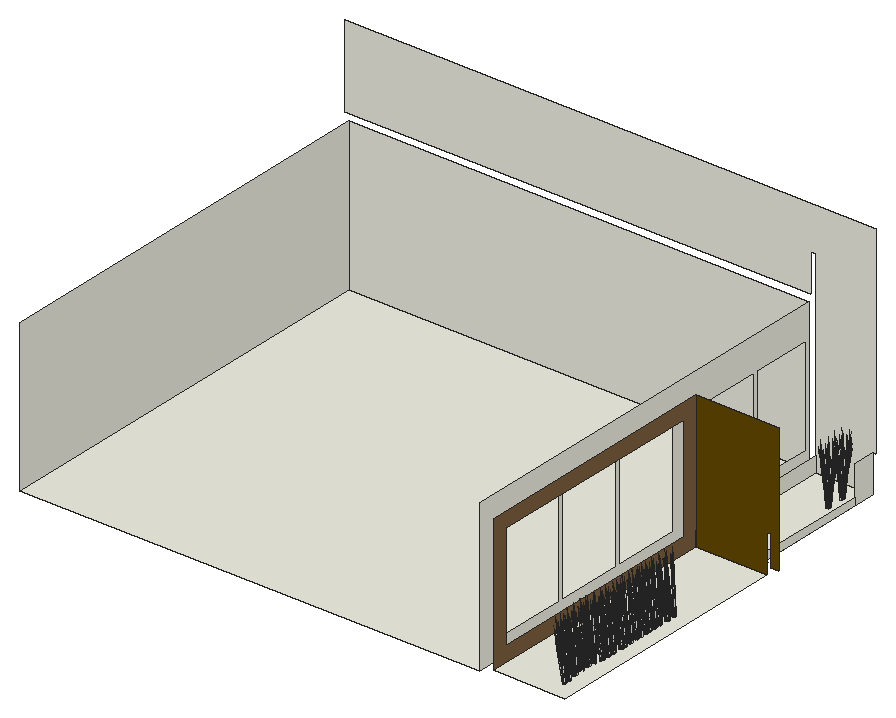
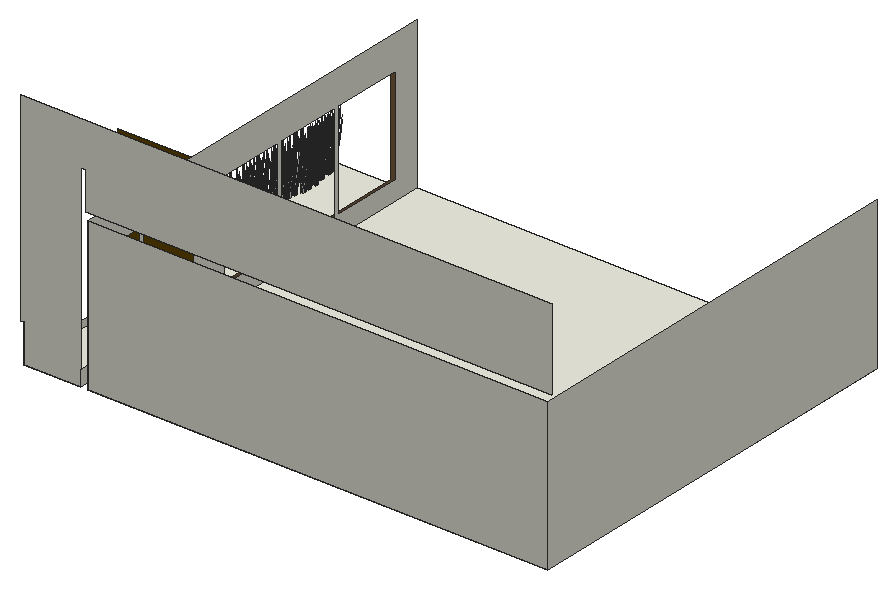
# SketchUp Ruby script. Lengths in inches.
U = 1.inch
M = Sketchup.active_model
def pt(a) = Geom::Point3d.new(a.map { |v| v * U })
def face(e, loops, mat)
  f = e.add_face(loops[0].map { |a| pt(a) })
  loops[1..].each { |l| e.add_face(l.map { |a| pt(a) }).erase! }
  f.material = f.back_material = mat if mat
  f
end
# faces: each face lists its corners as indices into pts; further lists are holes
def faces(e, pts, list, mat = nil) = list.each { |f| face(e, (f[0].is_a?(Array) ? f : [f]).map { |l| l.map { |i| pts[i] } }, mat) }
# xy, xz, yz: faces in a plane at the given z, y or x. An outline is a flat list of corners, or four numbers for a rectangle; further outlines are holes
def ring(l) = l.size == 4 ? [[l[0], l[1]], [l[2], l[1]], [l[2], l[3]], [l[0], l[3]]] : l.each_slice(2).to_a
def flat(e, list, mat, &to3) = list.each { |f| face(e, (f[0].is_a?(Array) ? f : [f]).map { |l| ring(l).map { |u, v| to3.(u, v) } }, mat) }
def xy(e, z, list, mat = nil) = flat(e, list, mat) { |x, y| [x, y, z] }
def xz(e, y, list, mat = nil) = flat(e, list, mat) { |x, z| [x, y, z] }
def yz(e, x, list, mat = nil) = flat(e, list, mat) { |y, z| [x, y, z] }
def lines(e, pts, list) = list.each { |a, b| e.add_line(pt(pts[a]), pt(pts[b])) }
# prism: a flat outline (further loops are holes) pulled along v
def prism(e, loops, v, mat = nil)
  f = face(e, loops, mat); d = Geom::Vector3d.new(v.map { |x| x * U })
  f.pushpull(f.normal.samedirection?(d) ? d.length : -d.length)
end
def box(e, o, s, mat = nil) = prism(e, [[o, [o[0] + s[0], o[1], o[2]], [o[0] + s[0], o[1] + s[1], o[2]], [o[0], o[1] + s[1], o[2]]]], [0, 0, s[2]], mat)
def at(x, y, z, deg = 0) = Geom::Transformation.translation(pt([x, y, z])) * Geom::Transformation.rotation(ORIGIN, Z_AXIS, deg.degrees)
def axes(o, x, y, z) = Geom::Transformation.new([*x, 0, *y, 0, *z, 0, *pt(o).to_a, 1])
def part(name) = M.definitions.add(name)
# library, detail: a bought-in or finely detailed component or shape, given as its bounding box
def library(name, o, s) = part(name).tap { |d| box(d.entities, o, s) }
def detail(e, o, s) = box(e.add_group.entities, o, s)
def put(e, d, t, mat = nil) = e.add_instance(d, t).tap { |i| i.material = mat if mat }
def group(e, t, mat = nil) = e.add_group.tap { |g| g.transformation = t; g.material = mat if mat }.entities
root = M.entities
M.materials.add("D01_Frost_White").color = [238, 238, 227]
M.materials.add("D08_Bronzed_Mustard").color = [102, 74, 0]
M.materials.add("LightPink_Translucent").color = [144, 107, 117]
M.materials["LightPink_Translucent"].alpha = 0.75
M.materials.add("Plywood_01_1K").color = [125, 96, 64]
c1 = part("blade")
p = [[2.15,0.21,22],[0,0.17,0],[0.09,0.45,0],[2.18,0.31,22],[2.29,0.31,22],[0.38,0.45,0],
  [2.48,0.24,33],[2.49,0.24,33],[2.48,0.22,33]]
faces(c1.entities,p,[[0,1,2,3],[4,5,2,3],[6,3,4,7],[8,0,3,6]])
c2 = part("seeds")
p = [[0.3,-0.1,1.38],[-0.01,-0.03,1.59],[-0.01,-0.03,0.03],[0.14,-0.07,-0.07],[0.29,-0.03,3],[0.15,0.01,3.11]]
faces(c2.entities,p,[[0,1,2,3],[1,0,4,5]],"LightPink_Translucent")
c3 = part("blade with seeds")
put(c3.entities,c1,at(0,0,0))
put(c3.entities,c2,axes([2.4,0.25,30.99],[1.5799,-0.05474,1.17369],[-0.12525,1.92788,0.29478],[-0.07173,-0.02425,1.56792]))
xy(root,150,[[10,367,376,694],[382,373,439,574.02],[382,574.02,430,586],[382,586,427,694]],"D01_Frost_White")
xz(root,574.02,[[382,150,439,150,439,180,442,180,442,156,448,156,448,258,382,258]],"D08_Bronzed_Mustard")
xz(root,694,[[382,150,427,150,427,180,430,180,430,341,7,341,7,276,377.5,276,377.5,306,382,306],[10,150,376,270]],"D01_Frost_White")
yz(root,10,[[367,150,694,270]],"D01_Frost_White")
yz(root,376,[[[367,150,694,270],[388,165,445.01,243],[505.01,165,559.02,243],[448.01,165,502.01,243],[589,165,640,243],[643,165,691,243]]],"D01_Frost_White")
yz(root,382,[[574.02,150,586,162],[586,150,694,162]],"D01_Frost_White")
yz(root,382,[[[373,150,574.02,258],[385,162,562.02,246]]],"Plywood_01_1K")
yz(root,427,[[586,150,676,156],[676,150,694,180]],"D01_Frost_White")
put(root,c3,axes([416.51,662.93,151.74],[-0.42629,-0.07733,-0.52676],[0.08996,-0.47699,-0.13825],[-0.12722,-0.0578,1.16273]))
put(root,c3,axes([416.51,676.81,151.74],[-0.42629,-0.07733,-0.52676],[0.08996,-0.47699,-0.13825],[-0.12722,-0.0578,1.16273]))
put(root,c3,axes([415.96,663.83,151.7],[-0.38354,-0.23583,-0.41945],[0.22925,-0.42288,0],[-0.08735,-0.05371,1.33059]))
put(root,c3,axes([415.96,677.71,151.7],[-0.38354,-0.23583,-0.41945],[0.22925,-0.42288,0],[-0.08735,-0.05371,1.33059]))
put(root,c3,axes([416.0625,663.66,151.71],[-0.09626,-0.41098,-0.2617],[0.38233,-0.1167,0.2617],[-0.07708,-0.04739,1.17405]))
put(root,c3,axes([416.0625,677.54,151.71],[-0.09626,-0.41098,-0.2617],[0.38233,-0.1167,0.2617],[-0.07708,-0.04739,1.17405]))
put(root,c3,axes([417.27,663.34,151.74],[-0.27603,0.35451,-0.52676],[-0.34289,-0.32147,-0.13825],[-0.11061,0.08844,1.16273]))
put(root,c3,axes([417.27,677.22,151.74],[-0.27603,0.35451,-0.52676],[-0.34289,-0.32147,-0.13825],[-0.11061,0.08844,1.16273]))
put(root,c3,axes([416.74,662.78,151.87],[-0.24618,-0.39589,-0.37796],[0.37289,-0.27878,0.1819],[-0.07967,-0.04899,1.2135]))
put(root,c3,axes([416.74,676.66,151.87],[-0.24618,-0.39589,-0.37796],[0.37289,-0.27878,0.1819],[-0.07967,-0.04899,1.2135]))
put(root,c3,axes([417.26,663.0625,151.87],[-0.44501,0.02912,-0.37796],[-0.04024,-0.48332,0.1819],[-0.07967,0.04899,1.2135]))
put(root,c3,axes([417.26,676.94,151.87],[-0.44501,0.02912,-0.37796],[-0.04024,-0.48332,0.1819],[-0.07967,0.04899,1.2135]))
put(root,c3,axes([417.73,664.3125,151.7],[-0.38354,0.23583,-0.41945],[-0.22925,-0.42288,0],[-0.08735,0.05371,1.33059]))
put(root,c3,axes([417.73,678.1875,151.7],[-0.38354,0.23583,-0.41945],[-0.22925,-0.42288,0],[-0.08735,0.05371,1.33059]))
put(root,c3,axes([415.46,661.96,151.7],[0,-0.47166,-0.41945],[0.45849,0,0],[0,-0.10742,1.33059]))
put(root,c3,axes([415.46,675.84,151.7],[0,-0.47166,-0.41945],[0.45849,0,0],[0,-0.10742,1.33059]))
put(root,c3,axes([417.64,664.125,151.71],[-0.38233,-0.1167,-0.2617],[0.09626,-0.41098,0.2617],[-0.07708,0.04739,1.17405]))
put(root,c3,axes([417.64,678,151.71],[-0.38233,-0.1167,-0.2617],[0.09626,-0.41098,0.2617],[-0.07708,0.04739,1.17405]))
put(root,c3,axes([416.45,662.03,151.77],[-0.1683,-0.48366,-0.58997],[0.48479,-0.17419,-0.15484],[-0.0186,-0.16378,1.30225]))
put(root,c3,axes([416.45,675.91,151.77],[-0.1683,-0.48366,-0.58997],[0.48479,-0.17419,-0.15484],[-0.0186,-0.16378,1.30225]))
put(root,c3,axes([415.65,661.97,151.71],[0.28606,-0.29428,-0.2617],[0.28606,0.29428,0.2617],[0,-0.09479,1.17405]))
put(root,c3,axes([415.65,675.85,151.71],[0.28606,-0.29428,-0.2617],[0.28606,0.29428,0.2617],[0,-0.09479,1.17405]))
put(root,c3,axes([416.7,662.15,151.87],[0.19883,-0.425,-0.37796],[0.41314,0.20454,0.1819],[0,-0.09797,1.2135]))
put(root,c3,axes([416.7,676.03,151.87],[0.19883,-0.425,-0.37796],[0.41314,0.20454,0.1819],[0,-0.09797,1.2135]))
put(root,c3,axes([417.75,662.72,151.87],[-0.19883,0.425,-0.37796],[-0.41314,-0.20454,0.1819],[0,0.09797,1.2135]))
put(root,c3,axes([417.75,676.6,151.87],[-0.19883,0.425,-0.37796],[-0.41314,-0.20454,0.1819],[0,0.09797,1.2135]))
put(root,c3,axes([418.8,662.9,151.71],[-0.28606,0.29428,-0.2617],[-0.28606,-0.29428,0.2617],[0,0.09479,1.17405]))
put(root,c3,axes([418.8,676.78,151.71],[-0.28606,0.29428,-0.2617],[-0.28606,-0.29428,0.2617],[0,0.09479,1.17405]))
put(root,c3,axes([417.99,662.85,151.77],[0.15027,0.43184,-0.5847],[-0.43285,0.15553,-0.15346],[0.01661,0.14623,1.29063]))
put(root,c3,axes([417.99,676.73,151.77],[0.15027,0.43184,-0.5847],[-0.43285,0.15553,-0.15346],[0.01661,0.14623,1.29063]))
put(root,c3,axes([416.82,660.75,151.71],[0.38233,0.1167,-0.2617],[-0.09626,0.41098,0.2617],[0.07708,-0.04739,1.17405]))
put(root,c3,axes([416.82,674.63,151.71],[0.38233,0.1167,-0.2617],[-0.09626,0.41098,0.2617],[0.07708,-0.04739,1.17405]))
put(root,c3,axes([419,662.92,151.7],[0,0.47166,-0.41945],[-0.45849,0,0],[0,0.10742,1.33059]))
put(root,c3,axes([419,676.79,151.7],[0,0.47166,-0.41945],[-0.45849,0,0],[0,0.10742,1.33059]))
put(root,c3,axes([416.73,660.57,151.7],[0.38354,-0.23583,-0.41945],[0.22925,0.42288,0],[0.08735,-0.05371,1.33059]))
put(root,c3,axes([416.73,674.44,151.7],[0.38354,-0.23583,-0.41945],[0.22925,0.42288,0],[0.08735,-0.05371,1.33059]))
put(root,c3,axes([417.72,662.1,151.87],[0.24618,0.39589,-0.37796],[-0.37289,0.27878,0.1819],[0.07967,0.04899,1.2135]))
put(root,c3,axes([417.72,675.97,151.87],[0.24618,0.39589,-0.37796],[-0.37289,0.27878,0.1819],[0.07967,0.04899,1.2135]))
put(root,c3,axes([417.19,661.53,151.74],[0.27603,-0.35451,-0.52676],[0.34289,0.32147,-0.13825],[0.11061,-0.08844,1.16273]))
put(root,c3,axes([417.19,675.41,151.74],[0.27603,-0.35451,-0.52676],[0.34289,0.32147,-0.13825],[0.11061,-0.08844,1.16273]))
put(root,c3,axes([418.4,661.22,151.71],[0.09626,0.41098,-0.2617],[-0.38233,0.1167,0.2617],[0.07708,0.04739,1.17405]))
put(root,c3,axes([418.4,675.1,151.71],[0.09626,0.41098,-0.2617],[-0.38233,0.1167,0.2617],[0.07708,0.04739,1.17405]))
put(root,c3,axes([418.5,661.04,151.7],[0.38354,0.23583,-0.41945],[-0.22925,0.42288,0],[0.08735,0.05371,1.33059]))
put(root,c3,axes([418.5,674.92,151.7],[0.38354,0.23583,-0.41945],[-0.22925,0.42288,0],[0.08735,0.05371,1.33059]))
put(root,c3,axes([417.94,661.95,151.74],[0.42629,0.07733,-0.52676],[-0.08996,0.47699,-0.13825],[0.12722,0.0578,1.16273]))
put(root,c3,axes([417.94,675.82,151.74],[0.42629,0.07733,-0.52676],[-0.08996,0.47699,-0.13825],[0.12722,0.0578,1.16273]))
put(root,c3,axes([426.07,405.04,151.74],[-0.42629,-0.07733,-0.52676],[0.08996,-0.47699,-0.13825],[-0.12722,-0.0578,1.16273]))
put(root,c3,axes([426.15,416.97,151.74],[-0.42629,-0.07733,-0.52676],[0.08996,-0.47699,-0.13825],[-0.12722,-0.0578,1.16273]))
put(root,c3,axes([426.22,411.59,151.74],[-0.42629,-0.07733,-0.52676],[0.08996,-0.47699,-0.13825],[-0.12722,-0.0578,1.16273]))
put(root,c3,axes([425.51,405.94,151.7],[-0.38354,-0.23583,-0.41945],[0.22925,-0.42288,0],[-0.08735,-0.05371,1.33059]))
put(root,c3,axes([425.59,417.875,151.7],[-0.38354,-0.23583,-0.41945],[0.22925,-0.42288,0],[-0.08735,-0.05371,1.33059]))
put(root,c3,axes([425.66,412.49,151.7],[-0.38354,-0.23583,-0.41945],[0.22925,-0.42288,0],[-0.08735,-0.05371,1.33059]))
put(root,c3,axes([425.62,405.77,151.71],[-0.09626,-0.41098,-0.2617],[0.38233,-0.1167,0.2617],[-0.07708,-0.04739,1.17405]))
put(root,c3,axes([425.69,417.7,151.71],[-0.09626,-0.41098,-0.2617],[0.38233,-0.1167,0.2617],[-0.07708,-0.04739,1.17405]))
put(root,c3,axes([427.16,397.46,151.74],[-0.42629,-0.07733,-0.52676],[0.08996,-0.47699,-0.13825],[-0.12722,-0.0578,1.16273]))
put(root,c3,axes([425.76,412.32,151.71],[-0.09626,-0.41098,-0.2617],[0.38233,-0.1167,0.2617],[-0.07708,-0.04739,1.17405]))
put(root,c3,axes([426.83,405.45,151.74],[-0.27603,0.35451,-0.52676],[-0.34289,-0.32147,-0.13825],[-0.11061,0.08844,1.16273]))
put(root,c3,axes([426.91,417.38,151.74],[-0.27603,0.35451,-0.52676],[-0.34289,-0.32147,-0.13825],[-0.11061,0.08844,1.16273]))
put(root,c3,axes([426.98,412,151.74],[-0.27603,0.35451,-0.52676],[-0.34289,-0.32147,-0.13825],[-0.11061,0.08844,1.16273]))
put(root,c3,axes([426.6,398.36,151.7],[-0.38354,-0.23583,-0.41945],[0.22925,-0.42288,0],[-0.08735,-0.05371,1.33059]))
put(root,c3,axes([426.29,404.89,151.87],[-0.24618,-0.39589,-0.37796],[0.37289,-0.27878,0.1819],[-0.07967,-0.04899,1.2135]))
put(root,c3,axes([426.37,416.82,151.87],[-0.24618,-0.39589,-0.37796],[0.37289,-0.27878,0.1819],[-0.07967,-0.04899,1.2135]))
put(root,c3,axes([426.4375,411.4375,151.87],[-0.24618,-0.39589,-0.37796],[0.37289,-0.27878,0.1819],[-0.07967,-0.04899,1.2135]))
put(root,c3,axes([426.82,405.17,151.87],[-0.44501,0.02912,-0.37796],[-0.04024,-0.48332,0.1819],[-0.07967,0.04899,1.2135]))
put(root,c3,axes([426.89,417.1,151.87],[-0.44501,0.02912,-0.37796],[-0.04024,-0.48332,0.1819],[-0.07967,0.04899,1.2135]))
put(root,c3,axes([426.96,411.72,151.87],[-0.44501,0.02912,-0.37796],[-0.04024,-0.48332,0.1819],[-0.07967,0.04899,1.2135]))
put(root,c3,axes([427.29,406.42,151.7],[-0.38354,0.23583,-0.41945],[-0.22925,-0.42288,0],[-0.08735,0.05371,1.33059]))
put(root,c3,axes([425.02,404.07,151.7],[0,-0.47166,-0.41945],[0.45849,0,0],[0,-0.10742,1.33059]))
put(root,c3,axes([427.36,418.35,151.7],[-0.38354,0.23583,-0.41945],[-0.22925,-0.42288,0],[-0.08735,0.05371,1.33059]))
put(root,c3,axes([425.09,416,151.7],[0,-0.47166,-0.41945],[0.45849,0,0],[0,-0.10742,1.33059]))
put(root,c3,axes([427.43,412.97,151.7],[-0.38354,0.23583,-0.41945],[-0.22925,-0.42288,0],[-0.08735,0.05371,1.33059]))
put(root,c3,axes([426.71,398.1875,151.71],[-0.09626,-0.41098,-0.2617],[0.38233,-0.1167,0.2617],[-0.07708,-0.04739,1.17405]))
put(root,c3,axes([425.16,410.62,151.7],[0,-0.47166,-0.41945],[0.45849,0,0],[0,-0.10742,1.33059]))
put(root,c3,axes([427.2,406.23,151.71],[-0.38233,-0.1167,-0.2617],[0.09626,-0.41098,0.2617],[-0.07708,0.04739,1.17405]))
put(root,c3,axes([427.27,418.16,151.71],[-0.38233,-0.1167,-0.2617],[0.09626,-0.41098,0.2617],[-0.07708,0.04739,1.17405]))
put(root,c3,axes([427.34,412.78,151.71],[-0.38233,-0.1167,-0.2617],[0.09626,-0.41098,0.2617],[-0.07708,0.04739,1.17405]))
put(root,c3,axes([427.92,397.875,151.74],[-0.27603,0.35451,-0.52676],[-0.34289,-0.32147,-0.13825],[-0.11061,0.08844,1.16273]))
put(root,c3,axes([426.01,404.14,151.77],[-0.1683,-0.48366,-0.58997],[0.48479,-0.17419,-0.15484],[-0.0186,-0.16378,1.30225]))
put(root,c3,axes([426.08,416.07,151.77],[-0.1683,-0.48366,-0.58997],[0.48479,-0.17419,-0.15484],[-0.0186,-0.16378,1.30225]))
put(root,c3,axes([428.51,384.47,151.74],[-0.42629,-0.07733,-0.52676],[0.08996,-0.47699,-0.13825],[-0.12722,-0.0578,1.16273]))
put(root,c3,axes([428.51,389.04,151.74],[-0.42629,-0.07733,-0.52676],[0.08996,-0.47699,-0.13825],[-0.12722,-0.0578,1.16273]))
put(root,c3,axes([428.51,423.125,151.74],[-0.42629,-0.07733,-0.52676],[0.08996,-0.47699,-0.13825],[-0.12722,-0.0578,1.16273]))
put(root,c3,axes([428.51,429.24,151.74],[-0.42629,-0.07733,-0.52676],[0.08996,-0.47699,-0.13825],[-0.12722,-0.0578,1.16273]))
put(root,c3,axes([428.51,434.15,151.74],[-0.42629,-0.07733,-0.52676],[0.08996,-0.47699,-0.13825],[-0.12722,-0.0578,1.16273]))
put(root,c3,axes([428.51,441.41,151.74],[-0.42629,-0.07733,-0.52676],[0.08996,-0.47699,-0.13825],[-0.12722,-0.0578,1.16273]))
put(root,c3,axes([428.51,445.1,151.74],[-0.42629,-0.07733,-0.52676],[0.08996,-0.47699,-0.13825],[-0.12722,-0.0578,1.16273]))
put(root,c3,axes([428.51,450.52,151.74],[-0.42629,-0.07733,-0.52676],[0.08996,-0.47699,-0.13825],[-0.12722,-0.0578,1.16273]))
put(root,c3,axes([428.51,457,151.74],[-0.42629,-0.07733,-0.52676],[0.08996,-0.47699,-0.13825],[-0.12722,-0.0578,1.16273]))
put(root,c3,axes([428.51,460.55,151.74],[-0.42629,-0.07733,-0.52676],[0.08996,-0.47699,-0.13825],[-0.12722,-0.0578,1.16273]))
put(root,c3,axes([428.51,465.95,151.74],[-0.42629,-0.07733,-0.52676],[0.08996,-0.47699,-0.13825],[-0.12722,-0.0578,1.16273]))
put(root,c3,axes([428.51,470.01,151.74],[-0.42629,-0.07733,-0.52676],[0.08996,-0.47699,-0.13825],[-0.12722,-0.0578,1.16273]))
put(root,c3,axes([428.51,474.33,151.74],[-0.42629,-0.07733,-0.52676],[0.08996,-0.47699,-0.13825],[-0.12722,-0.0578,1.16273]))
put(root,c3,axes([428.51,479.87,151.74],[-0.42629,-0.07733,-0.52676],[0.08996,-0.47699,-0.13825],[-0.12722,-0.0578,1.16273]))
put(root,c3,axes([428.51,487.08,151.74],[-0.42629,-0.07733,-0.52676],[0.08996,-0.47699,-0.13825],[-0.12722,-0.0578,1.16273]))
put(root,c3,axes([428.51,493.25,151.74],[-0.42629,-0.07733,-0.52676],[0.08996,-0.47699,-0.13825],[-0.12722,-0.0578,1.16273]))
put(root,c3,axes([427.38,397.31,151.87],[-0.24618,-0.39589,-0.37796],[0.37289,-0.27878,0.1819],[-0.07967,-0.04899,1.2135]))
put(root,c3,axes([426.15,410.6875,151.77],[-0.1683,-0.48366,-0.58997],[0.48479,-0.17419,-0.15484],[-0.0186,-0.16378,1.30225]))
put(root,c3,axes([425.21,404.08,151.71],[0.28606,-0.29428,-0.2617],[0.28606,0.29428,0.2617],[0,-0.09479,1.17405]))
put(root,c3,axes([425.29,416.01,151.71],[0.28606,-0.29428,-0.2617],[0.28606,0.29428,0.2617],[0,-0.09479,1.17405]))
put(root,c3,axes([427.9,397.59,151.87],[-0.44501,0.02912,-0.37796],[-0.04024,-0.48332,0.1819],[-0.07967,0.04899,1.2135]))
put(root,c3,axes([425.36,410.63,151.71],[0.28606,-0.29428,-0.2617],[0.28606,0.29428,0.2617],[0,-0.09479,1.17405]))
put(root,c3,axes([427.96,385.37,151.7],[-0.38354,-0.23583,-0.41945],[0.22925,-0.42288,0],[-0.08735,-0.05371,1.33059]))
put(root,c3,axes([427.96,389.9375,151.7],[-0.38354,-0.23583,-0.41945],[0.22925,-0.42288,0],[-0.08735,-0.05371,1.33059]))
put(root,c3,axes([427.96,424.03,151.7],[-0.38354,-0.23583,-0.41945],[0.22925,-0.42288,0],[-0.08735,-0.05371,1.33059]))
put(root,c3,axes([427.96,430.14,151.7],[-0.38354,-0.23583,-0.41945],[0.22925,-0.42288,0],[-0.08735,-0.05371,1.33059]))
put(root,c3,axes([427.96,435.05,151.7],[-0.38354,-0.23583,-0.41945],[0.22925,-0.42288,0],[-0.08735,-0.05371,1.33059]))
put(root,c3,axes([427.96,442.31,151.7],[-0.38354,-0.23583,-0.41945],[0.22925,-0.42288,0],[-0.08735,-0.05371,1.33059]))
put(root,c3,axes([427.96,446,151.7],[-0.38354,-0.23583,-0.41945],[0.22925,-0.42288,0],[-0.08735,-0.05371,1.33059]))
put(root,c3,axes([427.96,451.42,151.7],[-0.38354,-0.23583,-0.41945],[0.22925,-0.42288,0],[-0.08735,-0.05371,1.33059]))
put(root,c3,axes([427.96,457.91,151.7],[-0.38354,-0.23583,-0.41945],[0.22925,-0.42288,0],[-0.08735,-0.05371,1.33059]))
put(root,c3,axes([427.96,461.45,151.7],[-0.38354,-0.23583,-0.41945],[0.22925,-0.42288,0],[-0.08735,-0.05371,1.33059]))
put(root,c3,axes([427.96,466.86,151.7],[-0.38354,-0.23583,-0.41945],[0.22925,-0.42288,0],[-0.08735,-0.05371,1.33059]))
put(root,c3,axes([427.96,470.91,151.7],[-0.38354,-0.23583,-0.41945],[0.22925,-0.42288,0],[-0.08735,-0.05371,1.33059]))
put(root,c3,axes([427.96,475.23,151.7],[-0.38354,-0.23583,-0.41945],[0.22925,-0.42288,0],[-0.08735,-0.05371,1.33059]))
put(root,c3,axes([427.96,480.77,151.7],[-0.38354,-0.23583,-0.41945],[0.22925,-0.42288,0],[-0.08735,-0.05371,1.33059]))
put(root,c3,axes([427.96,487.98,151.7],[-0.38354,-0.23583,-0.41945],[0.22925,-0.42288,0],[-0.08735,-0.05371,1.33059]))
put(root,c3,axes([427.96,494.15,151.7],[-0.38354,-0.23583,-0.41945],[0.22925,-0.42288,0],[-0.08735,-0.05371,1.33059]))
put(root,c3,axes([428.37,398.84,151.7],[-0.38354,0.23583,-0.41945],[-0.22925,-0.42288,0],[-0.08735,0.05371,1.33059]))
put(root,c3,axes([426.1,396.49,151.7],[0,-0.47166,-0.41945],[0.45849,0,0],[0,-0.10742,1.33059]))
put(root,c3,axes([428.28,398.65,151.71],[-0.38233,-0.1167,-0.2617],[0.09626,-0.41098,0.2617],[-0.07708,0.04739,1.17405]))
put(root,c3,axes([428.0625,385.19,151.71],[-0.09626,-0.41098,-0.2617],[0.38233,-0.1167,0.2617],[-0.07708,-0.04739,1.17405]))
put(root,c3,axes([428.0625,389.76,151.71],[-0.09626,-0.41098,-0.2617],[0.38233,-0.1167,0.2617],[-0.07708,-0.04739,1.17405]))
put(root,c3,axes([428.0625,423.85,151.71],[-0.09626,-0.41098,-0.2617],[0.38233,-0.1167,0.2617],[-0.07708,-0.04739,1.17405]))
put(root,c3,axes([428.0625,429.97,151.71],[-0.09626,-0.41098,-0.2617],[0.38233,-0.1167,0.2617],[-0.07708,-0.04739,1.17405]))
put(root,c3,axes([428.0625,434.88,151.71],[-0.09626,-0.41098,-0.2617],[0.38233,-0.1167,0.2617],[-0.07708,-0.04739,1.17405]))
put(root,c3,axes([428.0625,442.13,151.71],[-0.09626,-0.41098,-0.2617],[0.38233,-0.1167,0.2617],[-0.07708,-0.04739,1.17405]))
put(root,c3,axes([428.0625,445.83,151.71],[-0.09626,-0.41098,-0.2617],[0.38233,-0.1167,0.2617],[-0.07708,-0.04739,1.17405]))
put(root,c3,axes([428.0625,451.25,151.71],[-0.09626,-0.41098,-0.2617],[0.38233,-0.1167,0.2617],[-0.07708,-0.04739,1.17405]))
put(root,c3,axes([428.0625,457.73,151.71],[-0.09626,-0.41098,-0.2617],[0.38233,-0.1167,0.2617],[-0.07708,-0.04739,1.17405]))
put(root,c3,axes([428.0625,461.28,151.71],[-0.09626,-0.41098,-0.2617],[0.38233,-0.1167,0.2617],[-0.07708,-0.04739,1.17405]))
put(root,c3,axes([428.0625,466.68,151.71],[-0.09626,-0.41098,-0.2617],[0.38233,-0.1167,0.2617],[-0.07708,-0.04739,1.17405]))
put(root,c3,axes([428.0625,470.73,151.71],[-0.09626,-0.41098,-0.2617],[0.38233,-0.1167,0.2617],[-0.07708,-0.04739,1.17405]))
put(root,c3,axes([428.0625,475.06,151.71],[-0.09626,-0.41098,-0.2617],[0.38233,-0.1167,0.2617],[-0.07708,-0.04739,1.17405]))
put(root,c3,axes([428.0625,480.59,151.71],[-0.09626,-0.41098,-0.2617],[0.38233,-0.1167,0.2617],[-0.07708,-0.04739,1.17405]))
put(root,c3,axes([428.0625,487.81,151.71],[-0.09626,-0.41098,-0.2617],[0.38233,-0.1167,0.2617],[-0.07708,-0.04739,1.17405]))
put(root,c3,axes([428.0625,493.97,151.71],[-0.09626,-0.41098,-0.2617],[0.38233,-0.1167,0.2617],[-0.07708,-0.04739,1.17405]))
put(root,c3,axes([427.09,396.56,151.77],[-0.1683,-0.48366,-0.58997],[0.48479,-0.17419,-0.15484],[-0.0186,-0.16378,1.30225]))
put(root,c3,axes([426.26,404.26,151.87],[0.19883,-0.425,-0.37796],[0.41314,0.20454,0.1819],[0,-0.09797,1.2135]))
put(root,c3,axes([426.34,416.19,151.87],[0.19883,-0.425,-0.37796],[0.41314,0.20454,0.1819],[0,-0.09797,1.2135]))
put(root,c3,axes([426.3,396.5,151.71],[0.28606,-0.29428,-0.2617],[0.28606,0.29428,0.2617],[0,-0.09479,1.17405]))
put(root,c3,axes([426.41,410.8125,151.87],[0.19883,-0.425,-0.37796],[0.41314,0.20454,0.1819],[0,-0.09797,1.2135]))
put(root,c3,axes([429.27,384.88,151.74],[-0.27603,0.35451,-0.52676],[-0.34289,-0.32147,-0.13825],[-0.11061,0.08844,1.16273]))
put(root,c3,axes([429.27,389.45,151.74],[-0.27603,0.35451,-0.52676],[-0.34289,-0.32147,-0.13825],[-0.11061,0.08844,1.16273]))
put(root,c3,axes([429.27,423.54,151.74],[-0.27603,0.35451,-0.52676],[-0.34289,-0.32147,-0.13825],[-0.11061,0.08844,1.16273]))
put(root,c3,axes([429.27,429.65,151.74],[-0.27603,0.35451,-0.52676],[-0.34289,-0.32147,-0.13825],[-0.11061,0.08844,1.16273]))
put(root,c3,axes([429.27,434.5625,151.74],[-0.27603,0.35451,-0.52676],[-0.34289,-0.32147,-0.13825],[-0.11061,0.08844,1.16273]))
put(root,c3,axes([429.27,441.82,151.74],[-0.27603,0.35451,-0.52676],[-0.34289,-0.32147,-0.13825],[-0.11061,0.08844,1.16273]))
put(root,c3,axes([429.27,445.51,151.74],[-0.27603,0.35451,-0.52676],[-0.34289,-0.32147,-0.13825],[-0.11061,0.08844,1.16273]))
put(root,c3,axes([429.27,450.93,151.74],[-0.27603,0.35451,-0.52676],[-0.34289,-0.32147,-0.13825],[-0.11061,0.08844,1.16273]))
put(root,c3,axes([429.27,457.42,151.74],[-0.27603,0.35451,-0.52676],[-0.34289,-0.32147,-0.13825],[-0.11061,0.08844,1.16273]))
put(root,c3,axes([429.27,460.96,151.74],[-0.27603,0.35451,-0.52676],[-0.34289,-0.32147,-0.13825],[-0.11061,0.08844,1.16273]))
put(root,c3,axes([429.27,466.37,151.74],[-0.27603,0.35451,-0.52676],[-0.34289,-0.32147,-0.13825],[-0.11061,0.08844,1.16273]))
put(root,c3,axes([429.27,470.42,151.74],[-0.27603,0.35451,-0.52676],[-0.34289,-0.32147,-0.13825],[-0.11061,0.08844,1.16273]))
put(root,c3,axes([429.27,474.74,151.74],[-0.27603,0.35451,-0.52676],[-0.34289,-0.32147,-0.13825],[-0.11061,0.08844,1.16273]))
put(root,c3,axes([429.27,480.28,151.74],[-0.27603,0.35451,-0.52676],[-0.34289,-0.32147,-0.13825],[-0.11061,0.08844,1.16273]))
put(root,c3,axes([429.27,487.49,151.74],[-0.27603,0.35451,-0.52676],[-0.34289,-0.32147,-0.13825],[-0.11061,0.08844,1.16273]))
put(root,c3,axes([429.27,493.66,151.74],[-0.27603,0.35451,-0.52676],[-0.34289,-0.32147,-0.13825],[-0.11061,0.08844,1.16273]))
put(root,c3,axes([427.3125,404.83,151.87],[-0.19883,0.425,-0.37796],[-0.41314,-0.20454,0.1819],[0,0.09797,1.2135]))
put(root,c3,axes([427.39,416.76,151.87],[-0.19883,0.425,-0.37796],[-0.41314,-0.20454,0.1819],[0,0.09797,1.2135]))
put(root,c3,axes([428.74,384.3125,151.87],[-0.24618,-0.39589,-0.37796],[0.37289,-0.27878,0.1819],[-0.07967,-0.04899,1.2135]))
put(root,c3,axes([428.74,388.88,151.87],[-0.24618,-0.39589,-0.37796],[0.37289,-0.27878,0.1819],[-0.07967,-0.04899,1.2135]))
put(root,c3,axes([428.74,422.98,151.87],[-0.24618,-0.39589,-0.37796],[0.37289,-0.27878,0.1819],[-0.07967,-0.04899,1.2135]))
put(root,c3,axes([428.74,429.09,151.87],[-0.24618,-0.39589,-0.37796],[0.37289,-0.27878,0.1819],[-0.07967,-0.04899,1.2135]))
put(root,c3,axes([428.74,434,151.87],[-0.24618,-0.39589,-0.37796],[0.37289,-0.27878,0.1819],[-0.07967,-0.04899,1.2135]))
put(root,c3,axes([428.74,441.26,151.87],[-0.24618,-0.39589,-0.37796],[0.37289,-0.27878,0.1819],[-0.07967,-0.04899,1.2135]))
put(root,c3,axes([428.74,444.95,151.87],[-0.24618,-0.39589,-0.37796],[0.37289,-0.27878,0.1819],[-0.07967,-0.04899,1.2135]))
put(root,c3,axes([428.74,450.37,151.87],[-0.24618,-0.39589,-0.37796],[0.37289,-0.27878,0.1819],[-0.07967,-0.04899,1.2135]))
put(root,c3,axes([428.74,456.85,151.87],[-0.24618,-0.39589,-0.37796],[0.37289,-0.27878,0.1819],[-0.07967,-0.04899,1.2135]))
put(root,c3,axes([428.74,460.4,151.87],[-0.24618,-0.39589,-0.37796],[0.37289,-0.27878,0.1819],[-0.07967,-0.04899,1.2135]))
put(root,c3,axes([428.74,465.8,151.87],[-0.24618,-0.39589,-0.37796],[0.37289,-0.27878,0.1819],[-0.07967,-0.04899,1.2135]))
put(root,c3,axes([428.74,469.85,151.87],[-0.24618,-0.39589,-0.37796],[0.37289,-0.27878,0.1819],[-0.07967,-0.04899,1.2135]))
put(root,c3,axes([428.74,474.18,151.87],[-0.24618,-0.39589,-0.37796],[0.37289,-0.27878,0.1819],[-0.07967,-0.04899,1.2135]))
put(root,c3,axes([428.74,479.72,151.87],[-0.24618,-0.39589,-0.37796],[0.37289,-0.27878,0.1819],[-0.07967,-0.04899,1.2135]))
put(root,c3,axes([428.74,486.93,151.87],[-0.24618,-0.39589,-0.37796],[0.37289,-0.27878,0.1819],[-0.07967,-0.04899,1.2135]))
put(root,c3,axes([428.74,493.1,151.87],[-0.24618,-0.39589,-0.37796],[0.37289,-0.27878,0.1819],[-0.07967,-0.04899,1.2135]))
put(root,c3,axes([427.46,411.38,151.87],[-0.19883,0.425,-0.37796],[-0.41314,-0.20454,0.1819],[0,0.09797,1.2135]))
put(root,c3,axes([429.26,384.6,151.87],[-0.44501,0.02912,-0.37796],[-0.04024,-0.48332,0.1819],[-0.07967,0.04899,1.2135]))
put(root,c3,axes([429.26,389.17,151.87],[-0.44501,0.02912,-0.37796],[-0.04024,-0.48332,0.1819],[-0.07967,0.04899,1.2135]))
put(root,c3,axes([429.26,423.26,151.87],[-0.44501,0.02912,-0.37796],[-0.04024,-0.48332,0.1819],[-0.07967,0.04899,1.2135]))
put(root,c3,axes([429.26,429.37,151.87],[-0.44501,0.02912,-0.37796],[-0.04024,-0.48332,0.1819],[-0.07967,0.04899,1.2135]))
put(root,c3,axes([429.26,434.28,151.87],[-0.44501,0.02912,-0.37796],[-0.04024,-0.48332,0.1819],[-0.07967,0.04899,1.2135]))
put(root,c3,axes([429.26,441.54,151.87],[-0.44501,0.02912,-0.37796],[-0.04024,-0.48332,0.1819],[-0.07967,0.04899,1.2135]))
put(root,c3,axes([429.26,445.23,151.87],[-0.44501,0.02912,-0.37796],[-0.04024,-0.48332,0.1819],[-0.07967,0.04899,1.2135]))
put(root,c3,axes([429.26,450.65,151.87],[-0.44501,0.02912,-0.37796],[-0.04024,-0.48332,0.1819],[-0.07967,0.04899,1.2135]))
put(root,c3,axes([429.26,457.14,151.87],[-0.44501,0.02912,-0.37796],[-0.04024,-0.48332,0.1819],[-0.07967,0.04899,1.2135]))
put(root,c3,axes([429.26,460.68,151.87],[-0.44501,0.02912,-0.37796],[-0.04024,-0.48332,0.1819],[-0.07967,0.04899,1.2135]))
put(root,c3,axes([429.26,466.09,151.87],[-0.44501,0.02912,-0.37796],[-0.04024,-0.48332,0.1819],[-0.07967,0.04899,1.2135]))
put(root,c3,axes([429.26,470.14,151.87],[-0.44501,0.02912,-0.37796],[-0.04024,-0.48332,0.1819],[-0.07967,0.04899,1.2135]))
put(root,c3,axes([429.26,474.46,151.87],[-0.44501,0.02912,-0.37796],[-0.04024,-0.48332,0.1819],[-0.07967,0.04899,1.2135]))
put(root,c3,axes([429.26,480,151.87],[-0.44501,0.02912,-0.37796],[-0.04024,-0.48332,0.1819],[-0.07967,0.04899,1.2135]))
put(root,c3,axes([429.26,487.21,151.87],[-0.44501,0.02912,-0.37796],[-0.04024,-0.48332,0.1819],[-0.07967,0.04899,1.2135]))
put(root,c3,axes([429.26,493.38,151.87],[-0.44501,0.02912,-0.37796],[-0.04024,-0.48332,0.1819],[-0.07967,0.04899,1.2135]))
put(root,c3,axes([429.73,385.85,151.7],[-0.38354,0.23583,-0.41945],[-0.22925,-0.42288,0],[-0.08735,0.05371,1.33059]))
put(root,c3,axes([429.73,390.42,151.7],[-0.38354,0.23583,-0.41945],[-0.22925,-0.42288,0],[-0.08735,0.05371,1.33059]))
put(root,c3,axes([429.73,424.51,151.7],[-0.38354,0.23583,-0.41945],[-0.22925,-0.42288,0],[-0.08735,0.05371,1.33059]))
put(root,c3,axes([429.73,430.62,151.7],[-0.38354,0.23583,-0.41945],[-0.22925,-0.42288,0],[-0.08735,0.05371,1.33059]))
put(root,c3,axes([429.73,435.53,151.7],[-0.38354,0.23583,-0.41945],[-0.22925,-0.42288,0],[-0.08735,0.05371,1.33059]))
put(root,c3,axes([429.73,442.79,151.7],[-0.38354,0.23583,-0.41945],[-0.22925,-0.42288,0],[-0.08735,0.05371,1.33059]))
put(root,c3,axes([429.73,446.48,151.7],[-0.38354,0.23583,-0.41945],[-0.22925,-0.42288,0],[-0.08735,0.05371,1.33059]))
put(root,c3,axes([429.73,451.9,151.7],[-0.38354,0.23583,-0.41945],[-0.22925,-0.42288,0],[-0.08735,0.05371,1.33059]))
put(root,c3,axes([429.73,458.38,151.7],[-0.38354,0.23583,-0.41945],[-0.22925,-0.42288,0],[-0.08735,0.05371,1.33059]))
put(root,c3,axes([429.73,461.93,151.7],[-0.38354,0.23583,-0.41945],[-0.22925,-0.42288,0],[-0.08735,0.05371,1.33059]))
put(root,c3,axes([429.73,467.33,151.7],[-0.38354,0.23583,-0.41945],[-0.22925,-0.42288,0],[-0.08735,0.05371,1.33059]))
put(root,c3,axes([429.73,471.39,151.7],[-0.38354,0.23583,-0.41945],[-0.22925,-0.42288,0],[-0.08735,0.05371,1.33059]))
put(root,c3,axes([429.73,475.71,151.7],[-0.38354,0.23583,-0.41945],[-0.22925,-0.42288,0],[-0.08735,0.05371,1.33059]))
put(root,c3,axes([429.73,481.25,151.7],[-0.38354,0.23583,-0.41945],[-0.22925,-0.42288,0],[-0.08735,0.05371,1.33059]))
put(root,c3,axes([429.73,488.46,151.7],[-0.38354,0.23583,-0.41945],[-0.22925,-0.42288,0],[-0.08735,0.05371,1.33059]))
put(root,c3,axes([429.73,494.625,151.7],[-0.38354,0.23583,-0.41945],[-0.22925,-0.42288,0],[-0.08735,0.05371,1.33059]))
put(root,c3,axes([427.46,388.07,151.7],[0,-0.47166,-0.41945],[0.45849,0,0],[0,-0.10742,1.33059]))
put(root,c3,axes([427.46,422.16,151.7],[0,-0.47166,-0.41945],[0.45849,0,0],[0,-0.10742,1.33059]))
put(root,c3,axes([427.46,428.27,151.7],[0,-0.47166,-0.41945],[0.45849,0,0],[0,-0.10742,1.33059]))
put(root,c3,axes([427.46,433.18,151.7],[0,-0.47166,-0.41945],[0.45849,0,0],[0,-0.10742,1.33059]))
put(root,c3,axes([427.46,440.4375,151.7],[0,-0.47166,-0.41945],[0.45849,0,0],[0,-0.10742,1.33059]))
put(root,c3,axes([427.46,444.13,151.7],[0,-0.47166,-0.41945],[0.45849,0,0],[0,-0.10742,1.33059]))
put(root,c3,axes([427.46,449.55,151.7],[0,-0.47166,-0.41945],[0.45849,0,0],[0,-0.10742,1.33059]))
put(root,c3,axes([427.46,456.03,151.7],[0,-0.47166,-0.41945],[0.45849,0,0],[0,-0.10742,1.33059]))
put(root,c3,axes([427.46,459.58,151.7],[0,-0.47166,-0.41945],[0.45849,0,0],[0,-0.10742,1.33059]))
put(root,c3,axes([427.46,464.98,151.7],[0,-0.47166,-0.41945],[0.45849,0,0],[0,-0.10742,1.33059]))
put(root,c3,axes([427.46,469.04,151.7],[0,-0.47166,-0.41945],[0.45849,0,0],[0,-0.10742,1.33059]))
put(root,c3,axes([427.46,473.36,151.7],[0,-0.47166,-0.41945],[0.45849,0,0],[0,-0.10742,1.33059]))
put(root,c3,axes([427.46,478.9,151.7],[0,-0.47166,-0.41945],[0.45849,0,0],[0,-0.10742,1.33059]))
put(root,c3,axes([427.46,486.11,151.7],[0,-0.47166,-0.41945],[0.45849,0,0],[0,-0.10742,1.33059]))
put(root,c3,axes([427.46,492.28,151.7],[0,-0.47166,-0.41945],[0.45849,0,0],[0,-0.10742,1.33059]))
put(root,c3,axes([429.64,385.66,151.71],[-0.38233,-0.1167,-0.2617],[0.09626,-0.41098,0.2617],[-0.07708,0.04739,1.17405]))
put(root,c3,axes([429.64,390.23,151.71],[-0.38233,-0.1167,-0.2617],[0.09626,-0.41098,0.2617],[-0.07708,0.04739,1.17405]))
put(root,c3,axes([429.64,424.32,151.71],[-0.38233,-0.1167,-0.2617],[0.09626,-0.41098,0.2617],[-0.07708,0.04739,1.17405]))
put(root,c3,axes([429.64,430.43,151.71],[-0.38233,-0.1167,-0.2617],[0.09626,-0.41098,0.2617],[-0.07708,0.04739,1.17405]))
put(root,c3,axes([429.64,435.35,151.71],[-0.38233,-0.1167,-0.2617],[0.09626,-0.41098,0.2617],[-0.07708,0.04739,1.17405]))
put(root,c3,axes([429.64,442.6,151.71],[-0.38233,-0.1167,-0.2617],[0.09626,-0.41098,0.2617],[-0.07708,0.04739,1.17405]))
put(root,c3,axes([429.64,446.29,151.71],[-0.38233,-0.1167,-0.2617],[0.09626,-0.41098,0.2617],[-0.07708,0.04739,1.17405]))
put(root,c3,axes([429.64,451.71,151.71],[-0.38233,-0.1167,-0.2617],[0.09626,-0.41098,0.2617],[-0.07708,0.04739,1.17405]))
put(root,c3,axes([429.64,458.2,151.71],[-0.38233,-0.1167,-0.2617],[0.09626,-0.41098,0.2617],[-0.07708,0.04739,1.17405]))
put(root,c3,axes([429.64,461.74,151.71],[-0.38233,-0.1167,-0.2617],[0.09626,-0.41098,0.2617],[-0.07708,0.04739,1.17405]))
put(root,c3,axes([429.64,467.15,151.71],[-0.38233,-0.1167,-0.2617],[0.09626,-0.41098,0.2617],[-0.07708,0.04739,1.17405]))
put(root,c3,axes([429.64,471.2,151.71],[-0.38233,-0.1167,-0.2617],[0.09626,-0.41098,0.2617],[-0.07708,0.04739,1.17405]))
put(root,c3,axes([429.64,475.53,151.71],[-0.38233,-0.1167,-0.2617],[0.09626,-0.41098,0.2617],[-0.07708,0.04739,1.17405]))
put(root,c3,axes([429.64,481.0625,151.71],[-0.38233,-0.1167,-0.2617],[0.09626,-0.41098,0.2617],[-0.07708,0.04739,1.17405]))
put(root,c3,axes([429.64,488.27,151.71],[-0.38233,-0.1167,-0.2617],[0.09626,-0.41098,0.2617],[-0.07708,0.04739,1.17405]))
put(root,c3,axes([429.64,494.44,151.71],[-0.38233,-0.1167,-0.2617],[0.09626,-0.41098,0.2617],[-0.07708,0.04739,1.17405]))
put(root,c3,axes([427.35,396.68,151.87],[0.19883,-0.425,-0.37796],[0.41314,0.20454,0.1819],[0,-0.09797,1.2135]))
put(root,c3,axes([428.36,405.01,151.71],[-0.28606,0.29428,-0.2617],[-0.28606,-0.29428,0.2617],[0,0.09479,1.17405]))
put(root,c3,axes([428.4375,416.94,151.71],[-0.28606,0.29428,-0.2617],[-0.28606,-0.29428,0.2617],[0,0.09479,1.17405]))
put(root,c3,axes([428.45,388.13,151.77],[-0.1683,-0.48366,-0.58997],[0.48479,-0.17419,-0.15484],[-0.0186,-0.16378,1.30225]))
put(root,c3,axes([428.45,422.22,151.77],[-0.1683,-0.48366,-0.58997],[0.48479,-0.17419,-0.15484],[-0.0186,-0.16378,1.30225]))
put(root,c3,axes([428.45,428.34,151.77],[-0.1683,-0.48366,-0.58997],[0.48479,-0.17419,-0.15484],[-0.0186,-0.16378,1.30225]))
